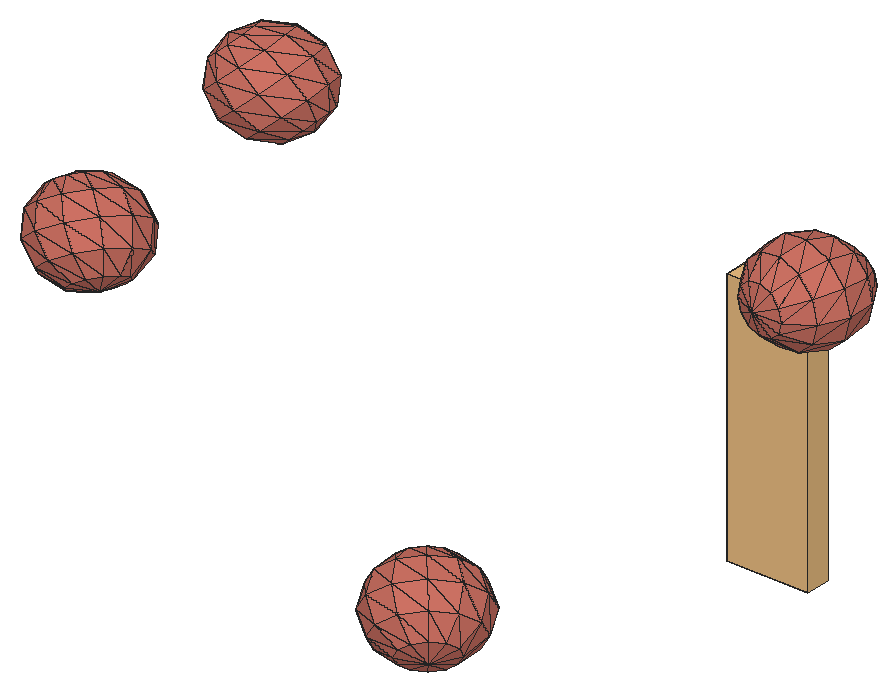
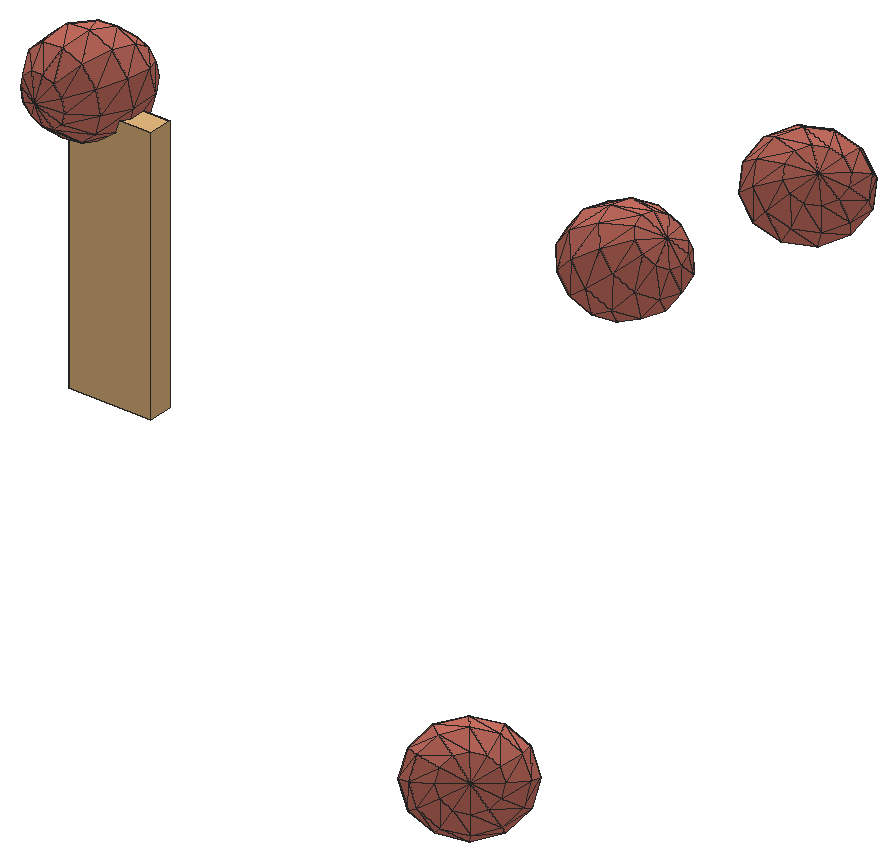
# SketchUp Ruby script. Lengths in inches.
U = 1.inch
M = Sketchup.active_model
def pt(a) = Geom::Point3d.new(a.map { |v| v * U })
def face(e, loops, mat)
  f = e.add_face(loops[0].map { |a| pt(a) })
  loops[1..].each { |l| e.add_face(l.map { |a| pt(a) }).erase! }
  f.material = f.back_material = mat if mat
  f
end
# faces: each face lists its corners as indices into pts; further lists are holes
def faces(e, pts, list, mat = nil) = list.each { |f| face(e, (f[0].is_a?(Array) ? f : [f]).map { |l| l.map { |i| pts[i] } }, mat) }
# xy, xz, yz: faces in a plane at the given z, y or x. An outline is a flat list of corners, or four numbers for a rectangle; further outlines are holes
def ring(l) = l.size == 4 ? [[l[0], l[1]], [l[2], l[1]], [l[2], l[3]], [l[0], l[3]]] : l.each_slice(2).to_a
def flat(e, list, mat, &to3) = list.each { |f| face(e, (f[0].is_a?(Array) ? f : [f]).map { |l| ring(l).map { |u, v| to3.(u, v) } }, mat) }
def xy(e, z, list, mat = nil) = flat(e, list, mat) { |x, y| [x, y, z] }
def xz(e, y, list, mat = nil) = flat(e, list, mat) { |x, z| [x, y, z] }
def yz(e, x, list, mat = nil) = flat(e, list, mat) { |y, z| [x, y, z] }
def lines(e, pts, list) = list.each { |a, b| e.add_line(pt(pts[a]), pt(pts[b])) }
# prism: a flat outline (further loops are holes) pulled along v
def prism(e, loops, v, mat = nil)
  f = face(e, loops, mat); d = Geom::Vector3d.new(v.map { |x| x * U })
  f.pushpull(f.normal.samedirection?(d) ? d.length : -d.length)
end
def box(e, o, s, mat = nil) = prism(e, [[o, [o[0] + s[0], o[1], o[2]], [o[0] + s[0], o[1] + s[1], o[2]], [o[0], o[1] + s[1], o[2]]]], [0, 0, s[2]], mat)
def at(x, y, z, deg = 0) = Geom::Transformation.translation(pt([x, y, z])) * Geom::Transformation.rotation(ORIGIN, Z_AXIS, deg.degrees)
def axes(o, x, y, z) = Geom::Transformation.new([*x, 0, *y, 0, *z, 0, *pt(o).to_a, 1])
def part(name) = M.definitions.add(name)
# library, detail: a bought-in or finely detailed component or shape, given as its bounding box
def library(name, o, s) = part(name).tap { |d| box(d.entities, o, s) }
def detail(e, o, s) = box(e.add_group.entities, o, s)
def put(e, d, t, mat = nil) = e.add_instance(d, t).tap { |i| i.material = mat if mat }
def group(e, t, mat = nil) = e.add_group.tap { |g| g.transformation = t; g.material = mat if mat }.entities
root = M.entities
M.materials.add("green").color = [174, 139, 102]
M.materials.add("vio").color = [206, 114, 100]
c1 = part("3DGeom~205_Defintion")
p = [[47.4,99.55,-486.18],[46.74,-121.12,-479.41],[-173.66,-85.23,-460.58],[170.15,120.28,-450.94],[-79.85,120.28,-475.32],[35.36,293.55,-362.6875],
  [33.56,-309.34,-344.18],[-220.94,-267.89,-322.44],[259.35,-85.23,-418.37],[-342.79,12.83,-366.9375],[-177.49,176.89,-421.25],[-416.23,-154.67,-214.3],
  [-416.23,-154.67,-214.3],[255.52,176.89,-379.03],[-415.33,146.77,-223.56],[-415.33,146.77,-223.56],[-219.38,254.22,-338.47],[279.06,-267.9,-273.69],
  [407.21,12.83,-293.82],[279.06,-267.9,-273.69],[259.35,-85.23,-418.37],[407.21,12.83,-293.82],[280.62,254.22,-289.72],[407.21,12.83,-293.82],
  [255.52,176.89,-379.03],[280.62,254.22,-289.72],[-342.79,12.83,-366.9375],[-416.23,-154.67,-214.3],[-500,0,-48.75],[-342.79,12.83,-366.9375],
  [-415.33,146.77,-223.56],[-194.27,331.56,-249.16],[238.74,331.56,-206.94],[-194.27,331.56,-249.16],[-108.91,388.17,-177.25],[35.36,293.55,-362.6875],
  [13.85,408.89,-142.01],[35.36,293.55,-362.6875],[141.09,388.17,-152.875],[35.36,293.55,-362.6875],[238.74,331.56,-206.94],[35.36,293.55,-362.6875],
  [33.56,-309.34,-344.18],[11.38,-414.67,-116.72],[-209.02,-378.78,-97.9],[279.06,-267.9,-273.69],[33.56,-309.34,-344.18],[33.56,-309.34,-344.18],
  [-209.02,-378.78,-97.9],[-220.94,-267.89,-322.44],[-219.38,254.22,-338.47],[-371.85,280.72,-68.87],[-219.38,254.22,-338.47],[-371.85,280.72,-68.87],
  [-194.27,331.56,-249.16],[-220.94,-267.89,-322.44],[-209.02,-378.78,-97.9],[-378.15,-280.72,-4.25],[-220.94,-267.89,-322.44],[407.21,12.83,-293.82],
  [449.79,-154.67,-129.87],[279.06,-267.9,-273.69],[450.69,146.77,-139.125],[407.21,12.83,-293.82],[280.62,254.22,-289.72],[407.21,12.83,-293.82],
  [238.74,331.56,-206.94],[280.62,254.22,-289.72],[279.06,-267.9,-273.69],[223.99,-378.78,-55.68],[223.99,-378.78,-55.68],[279.06,-267.9,-273.69],
  [-371.85,280.72,-68.87],[-223.99,378.78,55.68],[-449.79,154.67,129.87],[-371.85,280.72,-68.87],[-450.69,-146.77,139.13],[238.74,331.56,-206.94],
  [378.15,280.72,4.25],[378.15,280.72,4.25],[238.74,331.56,-206.94],[-11.38,414.67,116.72],[209.02,378.78,97.9],[378.15,280.72,4.25],
  [500,0,48.75],[371.85,-280.72,68.87],[223.99,-378.78,-55.68],[-141.09,-388.17,152.875],[-209.02,-378.78,-97.9],[-13.85,-408.89,142.01],
  [-209.02,-378.78,-97.9],[-238.74,-331.56,206.94],[-209.02,-378.78,-97.9],[-238.74,-331.56,206.94],[-378.15,-280.72,-4.25],[-371.85,280.72,-68.87],
  [-279.06,267.9,273.69],[-371.85,280.72,-68.87],[-279.06,267.9,273.69],[-223.99,378.78,55.68],[108.91,-388.17,177.25],[371.85,-280.72,68.87],
  [-407.21,-12.83,293.82],[-238.74,-331.56,206.94],[-280.62,-254.22,289.72],[416.23,154.67,214.31],[209.02,378.78,97.9],[415.33,-146.77,223.56],
  [-279.06,267.9,273.69],[-33.56,309.34,344.18],[371.85,-280.72,68.87],[194.27,-331.56,249.16],[194.27,-331.56,249.16],[209.02,378.78,97.9],
  [220.94,267.89,322.44],[220.94,267.89,322.44],[220.94,267.89,322.44],[-259.35,85.23,418.37],[-259.35,85.23,418.37],[-279.06,267.9,273.69],
  [-255.52,-176.89,379.03],[-255.52,-176.89,379.03],[-35.36,-293.55,362.6875],[-238.74,-331.56,206.94],[-280.62,-254.22,289.72],[-238.74,-331.56,206.94],
  [-35.36,-293.55,362.6875],[342.79,-12.83,366.9375],[220.94,267.89,322.44],[342.79,-12.83,366.9375],[416.23,154.67,214.31],[219.38,-254.22,338.47],
  [194.27,-331.56,249.16],[342.79,-12.83,366.9375],[219.38,-254.22,338.47],[415.33,-146.77,223.56],[194.27,-331.56,249.16],[219.38,-254.22,338.47],
  [-35.36,-293.55,362.6875],[-279.06,267.9,273.69],[-259.35,85.23,418.37],[-46.74,121.12,479.41],[-279.06,267.9,273.69],[-33.56,309.34,344.18],
  [-255.52,-176.89,379.03],[-280.62,-254.22,289.72],[-35.36,-293.55,362.6875],[-407.21,-12.83,293.82],[-170.15,-120.28,450.94],[-407.21,-12.83,293.82],
  [220.94,267.89,322.44],[173.66,85.23,460.58],[342.79,-12.83,366.9375],[-33.56,309.34,344.18],[220.94,267.89,322.44],[219.38,-254.22,338.47],
  [177.49,-176.89,421.25],[-35.36,-293.55,362.6875],[342.79,-12.83,366.9375],[219.38,-254.22,338.47],[-33.56,309.34,344.18],[-35.36,-293.55,362.6875],
  [-47.4,-99.55,486.18],[-35.36,-293.55,362.6875],[79.85,-120.28,475.32],[-35.36,-293.55,362.6875],[-35.36,-293.55,362.6875],[342.79,-12.83,366.9375]]
faces(c1.entities,p,[[0,1,2],[3,1,0],[0,2,4],[0,4,5],[3,0,5],[1,6,7],[8,6,1],[1,7,2],
  [3,8,1],[4,2,9],[4,9,10],[4,10,5],[2,7,11],[2,12,9],[13,8,3],[13,3,5],
  [10,9,14],[10,15,16],[10,16,5],[8,17,6],[18,19,20],[13,21,8],[22,23,24],[25,13,5],
  [26,27,28],[29,28,30],[16,31,5],[32,25,5],[33,34,35],[34,36,37],[36,38,39],[38,40,41],
  [42,43,44],[45,43,46],[47,48,49],[50,30,51],[52,53,54],[55,56,57],[58,57,27],[59,60,61],
  [62,60,63],[64,62,65],[66,62,67],[68,69,43],[60,70,71],[33,72,73],[33,73,34],[30,28,74],
  [30,74,75],[27,57,76],[27,76,28],[77,78,62],[38,79,80],[34,73,81],[34,81,36],[38,82,83],
  [36,82,38],[36,81,82],[62,84,60],[78,84,62],[60,85,86],[84,85,60],[43,87,88],[43,89,87],
  [69,89,43],[90,87,91],[92,93,94],[95,74,96],[97,98,99],[69,100,89],[101,100,69],[28,76,102],
  [28,102,74],[57,103,104],[57,104,76],[78,105,84],[106,105,78],[84,107,85],[105,107,84],[73,108,109],
  [73,109,81],[110,111,100],[107,112,85],[113,114,105],[81,115,82],[81,109,116],[74,102,117],[74,118,119],
  [76,104,120],[76,121,102],[87,89,122],[89,100,122],[123,87,122],[100,111,122],[124,125,126],[105,127,107],
  [128,129,130],[107,131,132],[133,134,135],[136,137,138],[139,140,141],[142,141,143],[144,145,146],[147,144,148],
  [149,148,140],[150,151,152],[153,151,154],[155,156,157],[158,156,159],[160,141,151],[148,144,161],[162,148,163],
  [164,162,165],[156,164,166],[151,156,167],[140,148,162],[140,162,141],[151,164,156],[141,164,151],[141,162,164]],"vio")
c2 = part("3DGeom~245_Defintion")
p = [[84.59,12.79,-493.27],[7.47,-267.01,-389.5],[-107.54,-84.94,-478.67],[229.32,-154.15,-406.37],[223.5,146.29,-413.58],[-82.81,176.3,-448.01],
  [-2.61,253.375,-402],[-216.38,-308.31,-268.27],[-301.4,-120.72,-373.68],[-193.73,119.875,-439.57],[-228.02,292.57,-282.7],[-305.66,99.22,-378.96],
  [389.73,0,-314.35],[271.98,279.79,-260.94],[389.73,0,-314.35],[223.5,146.29,-413.58],[25.38,330.46,-313.87],[271.98,279.79,-260.94],
  [120.48,-377.52,-195.97],[312.61,-279.79,-210.57],[120.48,-377.52,-195.97],[389.73,0,-314.35],[312.61,-279.79,-210.57],[229.32,-154.15,-406.37],
  [7.47,-267.01,-389.5],[-73.38,-413.29,-90.98],[-216.38,-308.31,-268.27],[7.47,-267.01,-389.5],[120.48,-377.52,-195.97],[-305.66,99.22,-378.96],
  [-301.4,-120.72,-373.68],[-445.05,-84.94,-206.44],[-305.66,99.22,-378.96],[-388.6,119.875,-282.4],[-388.6,119.875,-282.4],[-301.4,-120.72,-373.68],
  [-216.38,-308.31,-268.27],[-382.26,-267.01,-75.16],[-301.4,-120.72,-373.68],[389.73,0,-314.35],[451.52,-146.29,-130.88],[312.61,-279.79,-210.57],
  [445.7,154.15,-138.1],[389.73,0,-314.35],[271.98,279.79,-260.94],[389.73,0,-314.35],[-6.34,386.88,-207.25],[271.98,279.79,-260.94],
  [25.38,330.46,-313.87],[25.38,330.46,-313.87],[-228.02,292.57,-282.7],[-420.32,176.3,-175.77],[-228.02,292.57,-282.7],[-392.33,253.375,-87.65],
  [-228.02,292.57,-282.7],[-312.13,330.46,-41.64],[-228.02,292.57,-282.7],[-312.13,330.46,-41.64],[-201.21,386.88,-50.07],[-228.02,292.57,-282.7],
  [-89.28,407.53,-110.6875],[-228.02,292.57,-282.7],[-228.02,292.57,-282.7],[-500,12.79,-21.75],[-216.38,-308.31,-268.27],[-217.03,-377.52,76.26],
  [-216.38,-308.31,-268.27],[-217.03,-377.52,76.26],[-382.26,-267.01,-75.16],[217.03,377.52,-76.26],[271.98,279.79,-260.94],[217.03,377.52,-76.26],
  [271.98,279.79,-260.94],[312.61,-279.79,-210.57],[201.21,-386.88,50.07],[312.61,-279.79,-210.57],[312.13,-330.46,41.64],[312.13,-330.46,41.64],
  [312.61,-279.79,-210.57],[-445.7,-154.15,138.1],[89.28,-407.53,110.6875],[-451.52,146.29,130.88],[500,-12.79,21.75],[382.26,267.01,75.16],
  [217.03,377.52,-76.26],[392.33,-253.375,87.65],[312.13,-330.46,41.64],[73.38,413.29,90.98],[6.34,-386.88,207.25],[-217.03,-377.52,76.26],
  [-312.61,279.79,210.57],[-312.61,279.79,210.57],[-312.13,330.46,-41.64],[382.26,267.01,75.16],[-217.03,-377.52,76.26],[-271.98,-279.79,260.94],
  [-120.48,377.52,195.97],[-312.61,279.79,210.57],[-389.73,0,314.35],[420.32,-176.3,175.78],[445.05,84.94,206.44],[228.02,-292.57,282.7],
  [312.13,-330.46,41.64],[228.02,-292.57,282.7],[216.38,308.31,268.27],[216.38,308.31,268.27],[382.26,267.01,75.16],[-217.03,-377.52,76.26],
  [-25.38,-330.46,313.87],[-217.03,-377.52,76.26],[-25.38,-330.46,313.87],[-271.98,-279.79,260.94],[228.02,-292.57,282.7],[-229.32,154.15,406.37],
  [-229.32,154.15,406.37],[-312.61,279.79,210.57],[-223.5,-146.29,413.58],[-223.5,-146.29,413.58],[388.6,-119.875,282.4],[228.02,-292.57,282.7],
  [-312.61,279.79,210.57],[-7.47,267.01,389.5],[-120.48,377.52,195.97],[-7.47,267.01,389.5],[301.4,120.72,373.68],[216.38,308.31,268.27],
  [-25.38,-330.46,313.87],[-312.61,279.79,210.57],[-229.32,154.15,406.37],[-7.47,267.01,389.5],[-271.98,-279.79,260.94],[-25.38,-330.46,313.87],
  [2.61,-253.375,402],[-271.98,-279.79,260.94],[-223.5,-146.29,413.58],[-7.47,267.01,389.5],[301.4,120.72,373.68],[216.38,308.31,268.27],
  [388.6,-119.875,282.4],[305.66,-99.22,378.96],[228.02,-292.57,282.7],[305.66,-99.22,378.96],[228.02,-292.57,282.7],[82.81,-176.3,448.01],
  [228.02,-292.57,282.7],[193.73,-119.875,439.57],[228.02,-292.57,282.7],[305.66,-99.22,378.96],[228.02,-292.57,282.7],[-389.73,0,314.35],
  [-84.59,-12.79,493.27],[-389.73,0,314.35],[107.54,84.94,478.67],[305.66,-99.22,378.96],[301.4,120.72,373.68],[-7.47,267.01,389.5],
  [301.4,120.72,373.68],[305.66,-99.22,378.96],[-7.47,267.01,389.5]]
faces(c2.entities,p,[[0,1,2],[0,3,1],[4,3,0],[5,0,2],[6,0,5],[6,4,0],[2,7,8],[2,1,7],
  [9,2,8],[5,2,9],[5,9,10],[6,5,10],[9,8,11],[9,11,10],[4,12,3],[13,14,15],
  [16,4,6],[16,17,4],[3,18,1],[3,19,20],[21,22,23],[16,6,10],[24,25,26],[27,28,25],
  [29,30,31],[32,31,33],[11,34,10],[35,36,37],[38,37,31],[39,40,41],[42,40,43],[44,42,45],
  [46,47,48],[46,49,50],[33,51,52],[51,53,54],[53,55,56],[57,58,59],[60,46,61],[58,60,62],
  [33,31,63],[33,63,51],[64,25,65],[66,67,68],[69,42,70],[46,71,72],[73,74,28],[75,76,74],
  [40,77,78],[60,71,46],[31,37,79],[31,79,63],[28,80,25],[28,74,80],[51,63,81],[51,81,53],
  [42,82,40],[83,82,42],[84,83,42],[40,85,86],[82,85,40],[60,87,71],[58,87,60],[25,88,89],
  [25,80,88],[53,81,90],[53,91,92],[87,93,71],[37,94,95],[37,95,79],[57,96,58],[58,96,87],
  [57,97,96],[63,79,98],[63,98,81],[82,99,85],[100,99,82],[83,100,82],[74,76,101],[102,85,103],
  [80,74,101],[104,100,83],[87,105,106],[107,88,108],[109,110,111],[85,99,112],[96,105,87],[88,80,101],
  [81,98,113],[81,114,115],[79,95,116],[79,117,98],[99,118,119],[100,118,99],[120,121,122],[96,123,105],
  [124,118,100],[125,124,100],[126,88,101],[127,128,129],[130,131,132],[133,132,134],[135,136,137],[138,139,140],
  [124,141,118],[132,131,142],[143,132,144],[145,143,146],[147,145,148],[149,134,150],[151,150,128],[152,153,154],
  [155,152,156],[152,145,157],[128,152,158],[134,132,143],[128,150,152],[134,143,150],[150,143,145],[150,145,152]],"vio")
c3 = part("3DGeom~202_Defintion")
p = [[2.15,-326.37,-327.67],[-168.31,-180.33,-426.3],[-6.92,-60.875,-500],[2.15,-326.37,-327.67],[188.51,-188.43,-412.77],[188.51,-188.43,-412.77],
  [110.74,102.31,-477.91],[-200.49,82.99,-453.25],[-132.5625,177.21,-440.5],[188.51,-188.43,-412.77],[324.36,0,-387.27],[324.36,0,-387.27],
  [153.12,265.49,-365.96],[-108.09,271.42,-375.87],[-108.09,271.42,-375.87],[153.12,265.49,-365.96],[-293.67,14.02,-410.7],[-340.34,204.62,-285.05],
  [-340.34,204.62,-285.05],[-108.09,271.42,-375.87],[-340.34,204.62,-285.05],[-184.79,-376.86,-154.77],[-330.2,-224.0625,-276.5625],[-184.79,-376.86,-154.77],
  [2.15,-326.37,-327.67],[-330.2,-224.0625,-276.5625],[172.03,-384.95,-141.25],[2.15,-326.37,-327.67],[188.51,-188.43,-412.77],[188.51,-188.43,-412.77],
  [333.43,-265.49,-214.95],[333.43,-265.49,-214.95],[188.51,-188.43,-412.77],[324.36,0,-387.27],[-330.2,-224.0625,-276.5625],[-387.14,-11.23,-324.25],
  [-293.67,14.02,-410.7],[-387.14,-11.23,-324.25],[-340.34,204.62,-285.05],[451.08,-102.31,-192.86],[373.3,188.43,-258],[324.36,0,-387.27],
  [153.12,265.49,-365.96],[373.3,188.43,-258],[-133.64,340.39,-276.66],[-108.09,271.42,-375.87],[-340.34,204.62,-285.05],[153.12,265.49,-365.96],
  [-108.09,271.42,-375.87],[-133.64,340.39,-276.66],[373.3,188.43,-258],[108.875,384.95,-194.14],[10.14,-428.68,8.49],[-184.79,-376.86,-154.77],
  [-449.22,-180.33,-90.91],[-330.2,-224.0625,-276.5625],[-455.85,14.02,-217.06],[-481.39,82.99,-117.86],[-456.93,177.2,-53.23],[-389,271.42,-40.48],
  [-295.82,340.39,-83.03],[-295.82,340.39,-83.03],[-202.35,365.63,-169.48],[-202.35,365.63,-169.48],[-340.34,204.62,-285.05],[-322.21,-326.37,59.6],
  [-184.79,-376.86,-154.77],[-322.21,-326.37,59.6],[493.46,60.875,-80.91],[322.21,326.37,-59.6],[373.3,188.43,-258],[322.21,326.37,-59.6],
  [-493.46,-60.875,80.91],[295.82,-340.39,83.03],[333.43,-265.49,-214.95],[295.82,-340.39,83.03],[333.43,-265.49,-214.95],[389,-271.42,40.48],
  [389,-271.42,40.48],[322.21,326.37,-59.6],[-10.14,428.68,-8.49],[456.93,-177.2,53.23],[-295.82,340.39,-83.03],[-108.875,-384.95,194.14],
  [-322.21,-326.37,59.6],[202.35,-365.63,169.48],[295.82,-340.39,83.03],[-451.08,102.31,192.86],[-373.3,-188.43,258],[-322.21,-326.37,59.6],
  [-373.3,-188.43,258],[-172.03,384.95,141.25],[-389,271.42,-40.48],[481.39,-82.99,117.86],[449.22,180.33,90.91],[184.79,376.86,154.77],
  [322.21,326.37,-59.6],[184.79,376.86,154.77],[-333.43,265.49,214.95],[-389,271.42,-40.48],[-333.43,265.49,214.95],[184.79,376.86,154.77],
  [133.64,-340.39,276.66],[295.82,-340.39,83.03],[340.34,-204.62,285.05],[340.34,-204.62,285.05],[340.34,-204.62,285.05],[-153.12,-265.49,365.96],
  [-373.3,-188.43,258],[-324.36,0,387.27],[-373.3,-188.43,258],[-324.36,0,387.27],[202.35,-365.63,169.48],[340.34,-204.62,285.05],
  [455.85,-14.02,217.07],[330.2,224.0625,276.5625],[184.79,376.86,154.77],[330.2,224.0625,276.5625],[340.34,-204.62,285.05],[-2.15,326.37,327.67],
  [-333.43,265.49,214.95],[184.79,376.86,154.77],[-2.15,326.37,327.67],[330.2,224.0625,276.5625],[184.79,376.86,154.77],[-2.15,326.37,327.67],
  [340.34,-204.62,285.05],[-188.51,188.43,412.77],[-324.36,0,387.27],[-188.51,188.43,412.77],[108.09,-271.42,375.87],[108.09,-271.42,375.87],
  [-2.15,326.37,327.67],[-333.43,265.49,214.95],[-188.51,188.43,412.77],[387.14,11.23,324.25],[340.34,-204.62,285.05],[330.2,224.0625,276.5625],
  [-110.74,-102.31,477.91],[-373.3,-188.43,258],[-153.12,-265.49,365.96],[-324.36,0,387.27],[-373.3,-188.43,258],[387.14,11.23,324.25],
  [168.31,180.33,426.3],[108.09,-271.42,375.87],[133.64,-340.39,276.66],[340.34,-204.62,285.05],[132.5625,-177.21,440.5],[340.34,-204.62,285.05],
  [200.49,-82.99,453.25],[340.34,-204.62,285.05],[293.67,-14.02,410.7],[340.34,-204.62,285.05],[293.67,-14.02,410.7],[340.34,-204.62,285.05],
  [387.14,11.23,324.25],[-188.51,188.43,412.77],[-153.12,-265.49,365.96],[-153.12,-265.49,365.96],[6.92,60.875,500]]
faces(c3.entities,p,[[0,1,2],[3,2,4],[5,2,6],[1,7,2],[2,7,8],[2,8,6],[9,6,10],[11,6,12],
  [6,8,13],[6,14,15],[1,16,7],[7,16,17],[8,7,18],[19,8,20],[21,22,1],[23,1,24],
  [25,16,1],[26,27,28],[26,29,30],[31,32,33],[34,35,16],[36,37,38],[31,33,39],[39,33,40],
  [41,42,43],[44,45,46],[47,48,49],[50,47,51],[47,49,51],[52,53,27],[52,27,26],[54,37,55],
  [54,56,37],[37,56,38],[56,57,38],[57,58,38],[58,59,38],[59,60,38],[61,62,38],[63,49,64],
  [51,49,63],[65,55,66],[67,54,55],[39,40,68],[68,40,69],[70,51,71],[72,56,54],[72,57,56],
  [73,26,74],[75,76,77],[78,31,39],[79,51,80],[51,63,80],[78,39,81],[81,39,68],[80,63,82],
  [83,53,52],[83,84,53],[85,52,26],[85,26,86],[87,57,72],[87,58,57],[88,54,89],[90,72,54],
  [91,82,92],[80,82,91],[81,68,93],[93,68,94],[68,69,94],[94,69,95],[96,80,97],[98,58,87],
  [98,59,58],[91,99,100],[101,80,91],[102,83,52],[102,52,85],[103,78,104],[78,81,105],[81,93,106],
  [107,84,83],[107,108,84],[109,72,110],[111,87,72],[112,103,113],[93,94,114],[114,94,115],[94,116,117],
  [93,114,118],[119,91,120],[121,91,122],[123,124,125],[102,85,126],[127,87,128],[129,98,87],[130,107,83],
  [131,83,102],[132,133,134],[114,135,136],[114,137,135],[138,139,140],[138,141,142],[143,123,144],[123,125,144],
  [145,146,147],[148,145,149],[150,148,151],[152,150,153],[135,154,155],[156,144,152],[144,125,157],[148,158,145],
  [148,138,159],[160,141,138],[160,157,141],[152,160,150],[152,144,160],[144,157,160],[150,138,148],[150,160,138]],"vio")
c4 = library("3DGeom~123_Defintion",[-47.43,-500,-158.67],[94.86,1000,317.34])
c5 = part("3DGeom~124_Defintion")
p = [[-44.78,-498.52,-137.32],[-32.6875,-500,-148.14],[-41.35,-495.57,-121.75],[-32.6875,-500,-148.14],[-44.78,-498.52,-137.32],[-40.2,-499.6,-144.3],
  [-41.35,-495.57,-121.75],[-32.6875,-500,-148.14],[-25.84,-494.09,-117],[-32.6875,-500,-148.14],[-24.26,-499.6,-147.81],[-17.18,-498.52,-143.39],
  [-13.75,-495.57,-127.82],[-32.6875,-500,-148.14],[-17.18,-498.52,-143.39],[-25.84,-494.09,-117],[-32.6875,-500,-148.14],[-13.75,-495.57,-127.82],
  [-13.75,-495.57,-127.82],[-17.18,-498.52,-143.39],[-13.33,-497.04,-136.08],[-44.78,-498.52,-137.32],[-41.35,-495.57,-121.75],[-45.2,-497.04,-129.06],
  [-25.84,-494.09,-117],[-13.75,-495.57,-127.82],[-18.33,-494.49,-120.84],[-41.35,-495.57,-121.75],[-25.84,-494.09,-117],[-34.27,-494.49,-117.33],
  [28.19,500,128.65],[26.39,491.3,158.41],[34.8,490.68,158.67],[28.19,500,128.65],[34.8,490.68,158.67],[42.32,491.3,154.91],
  [28.19,500,128.65],[19.34,493.01,154.2],[26.39,491.3,158.41],[28.19,500,128.65],[42.32,491.3,154.91],[46.95,493.01,148.13],
  [28.19,500,128.65],[15.56,495.34,147.17],[19.34,493.01,154.2],[28.19,500,128.65],[46.95,493.01,148.13],[47.43,495.34,140.16],
  [28.19,500,128.65],[16.04,497.67,139.19],[15.56,495.34,147.17],[28.19,500,128.65],[47.43,495.34,140.16],[43.65,497.67,133.12],
  [28.19,500,128.65],[20.67,499.375,132.42],[16.04,497.67,139.19],[28.19,500,128.65],[43.65,497.67,133.12],[36.61,499.375,128.91]]
faces(c5.entities,p,[[0,1,2],[3,4,5],[6,7,8],[9,10,11],[12,13,14],[15,16,17],[18,19,20],[21,22,23],
  [24,25,26],[27,28,29],[30,31,32],[33,34,35],[36,37,38],[39,40,41],[42,43,44],[45,46,47],
  [48,49,50],[51,52,53],[54,55,56],[57,58,59]],"green")
c6 = part("3DGeom~228_Defintion")
p = [[-95.24,-217.29,-433.01],[-345.24,0,-378.02],[-109.98,0,-500],[167.52,-188.18,-429.99],[154.76,0,-488],[-332.48,188.18,-320.01],
  [-95.24,217.29,-433.01],[385.39,-108.65,-311.75],[385.39,-108.65,-311.75],[378.02,0,-345.24],[167.52,188.18,-429.99],[378.02,0,-345.24],
  [-54.99,-376.36,-250],[-332.48,-188.18,-320.01],[202.38,-325.94,-271.5],[-297.62,325.94,-161.52],[-54.99,376.36,-250],[-297.62,325.94,-161.52],
  [-54.99,376.36,-250],[405.52,-188.18,-220.24],[405.52,-188.18,-220.24],[385.39,-108.65,-311.75],[378.02,0,-345.24],[385.39,108.65,-311.75],
  [385.39,108.65,-311.75],[202.38,325.94,-271.5],[-54.99,376.36,-250],[202.38,325.94,-271.5],[-332.48,-188.18,-320.01],[-488,0,-154.76],
  [-345.24,0,-378.02],[-345.24,0,-378.02],[-480.63,108.65,-121.26],[-345.24,0,-378.02],[-332.48,188.18,-320.01],[385.39,-108.65,-311.75],
  [378.02,0,-345.24],[500,0,-109.98],[385.39,108.65,-311.75],[-297.62,-325.94,-161.52],[-297.62,-325.94,-161.52],[-480.63,-108.65,-121.26],
  [-332.48,-188.18,-320.01],[-332.48,-188.18,-320.01],[-332.48,188.18,-320.01],[-460.51,188.18,-29.76],[-332.48,188.18,-320.01],[-297.62,325.94,-161.52],
  [405.52,-188.18,-220.24],[405.52,188.18,-220.24],[385.39,108.65,-311.75],[202.38,325.94,-271.5],[405.52,188.18,-220.24],[250,-376.36,-54.99],
  [-54.99,-376.36,-250],[202.38,-325.94,-271.5],[433.01,-217.29,-95.24],[250,-376.36,-54.99],[202.38,-325.94,-271.5],[202.38,-325.94,-271.5],
  [202.38,325.94,-271.5],[250,376.36,-54.99],[202.38,325.94,-271.5],[-54.99,376.36,-250],[0,434.59,0],[202.38,325.94,-271.5],
  [250,376.36,-54.99],[0,-434.59,0],[-297.62,-325.94,-161.52],[-54.99,-376.36,-250],[250,-376.36,-54.99],[-54.99,-376.36,-250],
  [-297.62,325.94,-161.52],[-250,376.36,54.99],[433.01,217.29,-95.24],[-250,-376.36,54.99],[-297.62,-325.94,-161.52],[-250,-376.36,54.99],
  [-460.51,-188.18,-29.76],[-297.62,-325.94,-161.52],[-297.62,-325.94,-161.52],[-297.62,325.94,-161.52],[-433.01,217.29,95.24],[-297.62,325.94,-161.52],
  [-250,376.36,54.99],[-500,0,109.98],[460.51,-188.18,29.76],[480.64,-108.65,121.26],[488,0,154.76],[460.51,188.18,29.76],
  [480.64,108.65,121.26],[297.625,325.94,161.52],[297.62,-325.94,161.52],[250,-376.36,-54.99],[297.62,-325.94,161.52],[250,376.36,-54.99],
  [54.99,376.36,250],[297.625,325.94,161.52],[250,376.36,-54.99],[54.99,376.36,250],[-250,-376.36,54.99],[-433.01,-217.29,95.24],
  [54.99,-376.36,250],[297.62,-325.94,161.52],[-202.375,325.94,271.5],[-202.375,325.94,271.5],[54.99,376.36,250],[332.49,188.18,320.01],
  [-202.38,-325.94,271.5],[-250,-376.36,54.99],[-202.38,-325.94,271.5],[-250,376.36,54.99],[-405.52,188.18,220.24],[-250,376.36,54.99],
  [-405.52,188.18,220.24],[-202.375,325.94,271.5],[-202.38,-325.94,271.5],[-405.52,-188.18,220.24],[-405.52,188.18,220.24],[-385.39,-108.65,311.75],
  [-385.39,-108.65,311.75],[-378.02,0,345.24],[-378.02,0,345.24],[-385.39,108.65,311.75],[-385.39,108.65,311.75],[-405.52,188.18,220.24],
  [332.48,-188.18,320.01],[345.24,0,378.02],[332.48,-188.18,320.01],[54.99,-376.36,250],[297.62,-325.94,161.52],[297.625,325.94,161.52],
  [95.25,217.29,433.01],[332.49,188.18,320.01],[297.625,325.94,161.52],[54.99,376.36,250],[-167.52,-188.18,429.99],[-405.52,-188.18,220.24],
  [-202.38,-325.94,271.5],[-385.39,-108.65,311.75],[-405.52,-188.18,220.24],[-202.375,325.94,271.5],[-405.52,188.18,220.24],[-385.39,108.65,311.75],
  [95.24,-217.29,433.01],[-202.38,-325.94,271.5],[54.99,-376.36,250],[332.48,-188.18,320.01],[54.99,-376.36,250],[-167.51,188.18,429.99],
  [-202.38,-325.94,271.5],[-154.76,0,488],[-378.02,0,345.24],[345.24,0,378.02],[332.48,-188.18,320.01],[332.49,188.18,320.01],
  [109.98,0,500],[332.49,188.18,320.01],[345.24,0,378.02],[345.24,0,378.02]]
faces(c6.entities,p,[[0,1,2],[3,0,2],[3,2,4],[2,1,5],[2,5,6],[4,2,6],[7,3,4],[8,4,9],
  [4,6,10],[11,4,10],[12,13,0],[14,12,0],[14,0,3],[0,13,1],[6,5,15],[10,6,16],
  [6,17,18],[19,14,3],[20,3,21],[22,10,23],[24,10,25],[10,26,27],[28,29,30],[31,29,32],
  [33,32,34],[35,36,37],[36,38,37],[12,39,13],[40,41,42],[43,41,29],[44,32,45],[46,45,47],
  [48,35,37],[38,49,37],[50,51,52],[53,54,55],[56,57,58],[56,59,48],[49,60,61],[62,63,64],
  [65,64,66],[67,68,69],[70,67,71],[63,72,73],[63,73,64],[56,48,37],[49,74,37],[49,61,74],
  [67,75,76],[77,78,79],[80,78,41],[81,45,82],[83,82,84],[29,41,85],[32,29,85],[41,78,85],
  [45,32,85],[86,56,37],[87,86,37],[88,87,37],[74,89,37],[89,90,37],[90,88,37],[86,57,56],
  [74,91,89],[74,61,91],[92,67,93],[86,94,57],[95,96,97],[98,64,99],[100,101,78],[78,101,85],
  [82,45,85],[102,75,67],[103,102,67],[64,73,104],[64,105,106],[87,94,86],[89,107,90],[89,91,107],
  [108,101,109],[102,110,75],[111,82,112],[113,114,115],[116,117,101],[101,117,85],[118,82,85],[117,119,85],
  [120,121,85],[122,123,85],[124,125,85],[87,126,94],[88,126,87],[90,107,127],[90,127,88],[88,127,126],
  [128,129,130],[131,132,133],[134,135,132],[136,137,138],[136,139,140],[141,142,143],[144,145,146],[147,144,148],
  [135,141,149],[135,149,132],[144,136,150],[141,143,149],[151,139,136],[151,152,139],[149,143,152],[153,144,154],
  [155,132,156],[157,156,158],[149,152,151],[159,156,144],[156,136,144],[156,151,136],[132,149,151],[132,151,156]],"vio")
g1 = group(root,at(15.3125,134.49,26.21))
put(g1,c1,axes([-0.58,0.38,11.37],[0,0.00039,0],[0,0,-0.00039],[-0.00039,0,0]),"vio")
g2 = group(root,at(15.3125,134.49,26.21))
put(g2,c2,axes([-0.58,-0.43,11.25],[0,0.00039,0],[0,0,-0.00039],[-0.00039,0,0]),"vio")
g3 = group(root,at(15.3125,134.49,26.21))
put(g3,c3,axes([-0.23,0.63,9.71],[0,0.00039,0],[0,0,-0.00039],[-0.00039,0,0]),"vio")
g4 = group(root,at(15.3125,134.49,26.21))
put(g4,c4,axes([1.13,0.48,10.83],[0,0.00091,0],[0,0,-0.00091],[-0.00091,0,0]),"green")
put(g4,c5,axes([1.13,0.48,10.83],[0,0.00091,0],[0,0,-0.00091],[-0.00091,0,0]),"green")
g5 = group(root,at(15.3125,134.49,26.21))
put(g5,c6,axes([1.26,0.45,11.32],[0,0.00038,0],[0,0,-0.00038],[-0.00038,0,0]),"vio")
